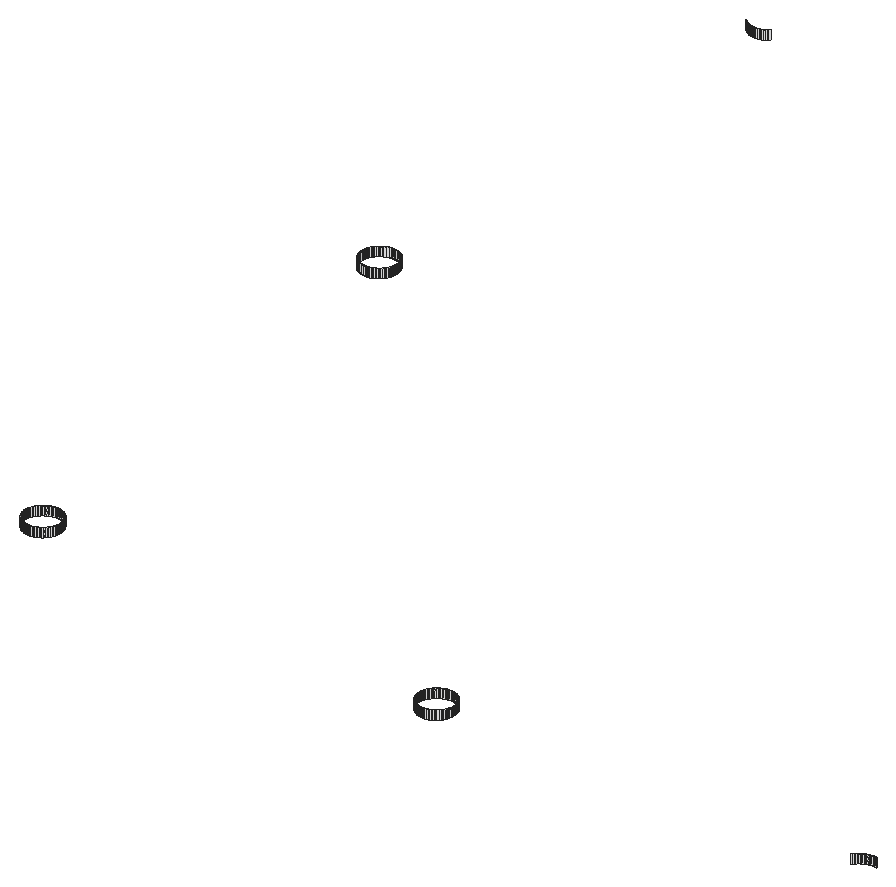
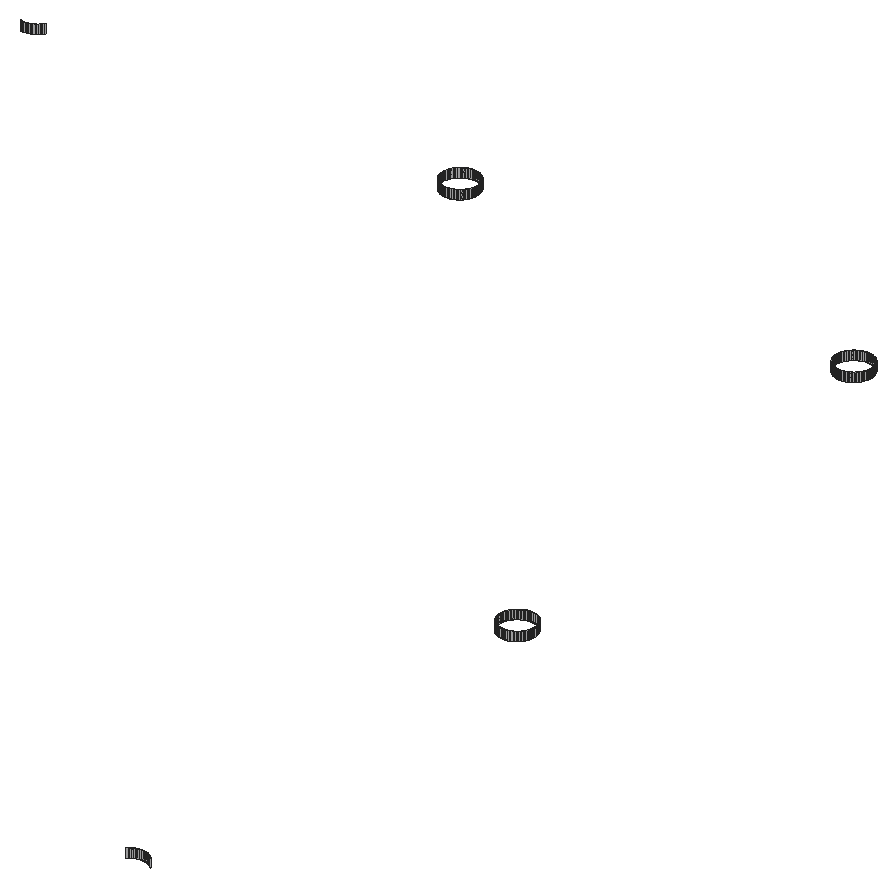
# SketchUp Ruby script. Lengths in inches.
U = 1.inch
M = Sketchup.active_model
def pt(a) = Geom::Point3d.new(a.map { |v| v * U })
def face(e, loops, mat)
  f = e.add_face(loops[0].map { |a| pt(a) })
  loops[1..].each { |l| e.add_face(l.map { |a| pt(a) }).erase! }
  f.material = f.back_material = mat if mat
  f
end
# faces: each face lists its corners as indices into pts; further lists are holes
def faces(e, pts, list, mat = nil) = list.each { |f| face(e, (f[0].is_a?(Array) ? f : [f]).map { |l| l.map { |i| pts[i] } }, mat) }
# xy, xz, yz: faces in a plane at the given z, y or x. An outline is a flat list of corners, or four numbers for a rectangle; further outlines are holes
def ring(l) = l.size == 4 ? [[l[0], l[1]], [l[2], l[1]], [l[2], l[3]], [l[0], l[3]]] : l.each_slice(2).to_a
def flat(e, list, mat, &to3) = list.each { |f| face(e, (f[0].is_a?(Array) ? f : [f]).map { |l| ring(l).map { |u, v| to3.(u, v) } }, mat) }
def xy(e, z, list, mat = nil) = flat(e, list, mat) { |x, y| [x, y, z] }
def xz(e, y, list, mat = nil) = flat(e, list, mat) { |x, z| [x, y, z] }
def yz(e, x, list, mat = nil) = flat(e, list, mat) { |y, z| [x, y, z] }
def lines(e, pts, list) = list.each { |a, b| e.add_line(pt(pts[a]), pt(pts[b])) }
# prism: a flat outline (further loops are holes) pulled along v
def prism(e, loops, v, mat = nil)
  f = face(e, loops, mat); d = Geom::Vector3d.new(v.map { |x| x * U })
  f.pushpull(f.normal.samedirection?(d) ? d.length : -d.length)
end
def box(e, o, s, mat = nil) = prism(e, [[o, [o[0] + s[0], o[1], o[2]], [o[0] + s[0], o[1] + s[1], o[2]], [o[0], o[1] + s[1], o[2]]]], [0, 0, s[2]], mat)
def at(x, y, z, deg = 0) = Geom::Transformation.translation(pt([x, y, z])) * Geom::Transformation.rotation(ORIGIN, Z_AXIS, deg.degrees)
def axes(o, x, y, z) = Geom::Transformation.new([*x, 0, *y, 0, *z, 0, *pt(o).to_a, 1])
def part(name) = M.definitions.add(name)
# library, detail: a bought-in or finely detailed component or shape, given as its bounding box
def library(name, o, s) = part(name).tap { |d| box(d.entities, o, s) }
def detail(e, o, s) = box(e.add_group.entities, o, s)
def put(e, d, t, mat = nil) = e.add_instance(d, t).tap { |i| i.material = mat if mat }
def group(e, t, mat = nil) = e.add_group.tap { |g| g.transformation = t; g.material = mat if mat }.entities
root = M.entities
M.materials.add("[Quartz Light Grey]").color = [251, 251, 252]
xz(root,52,[[86.9,111.81,87.02,112.81]],"[Quartz Light Grey]")
xz(root,56,[[38.9,111.81,39.02,112.81],[86.98,111.81,87.1,112.81],[134.98,111.81,135.1,112.81]],"[Quartz Light Grey]")
xz(root,60,[[38.98,111.81,39.1,112.81]],"[Quartz Light Grey]")
xz(root,115.35,[[32.85,111.81,32.98,112.81],[32.98,111.81,33.1,112.81]],"[Quartz Light Grey]")
xz(root,166.71,[[32.9,111.81,33.02,112.81],[33.02,111.81,33.15,112.81]],"[Quartz Light Grey]")
yz(root,31,[[113.33,111.81,113.46,112.81]],"[Quartz Light Grey]")
yz(root,35,[[113.25,111.81,113.375,112.81]],"[Quartz Light Grey]")
yz(root,37,[[57.98,111.81,58.1,112.81]],"[Quartz Light Grey]")
yz(root,41,[[57.9,111.81,58.02,112.81]],"[Quartz Light Grey]")
yz(root,85,[[53.98,111.81,54.1,112.81]],"[Quartz Light Grey]")
yz(root,89,[[53.9,111.81,54.02,112.81]],"[Quartz Light Grey]")
p = [[86.65,52.03,111.81],[86.52,52.06,111.81],[86.52,52.06,112.81],[86.65,52.03,112.81],[86.77,52.01,111.81],[86.77,52.01,112.81],
  [86.9,52,111.81],[86.9,52,112.81],[87.15,52.01,111.81],[87.02,52,111.81],[87.02,52,112.81],[87.15,52.01,112.81],
  [87.27,52.02,111.81],[87.27,52.02,112.81],[87.4,52.04,111.81],[87.4,52.04,112.81],[87.52,52.07,111.81],[87.52,52.07,112.81],
  [86.28,52.13,111.81],[86.17,52.18,111.81],[86.17,52.18,112.81],[86.28,52.13,112.81],[86.4,52.09,111.81],[86.4,52.09,112.81],
  [87.64,52.1,111.81],[87.64,52.1,112.81],[87.76,52.15,111.81],[87.76,52.15,112.81],[87.87,52.2,111.81],[87.87,52.2,112.81],
  [86.06,52.24,111.81],[85.95,52.3,111.81],[85.95,52.3,112.81],[86.06,52.24,112.81],[87.98,52.26,111.81],[87.98,52.26,112.81],
  [85.84,52.37,111.81],[85.84,52.37,112.81],[88.09,52.32,111.81],[88.09,52.32,112.81],[88.19,52.39,111.81],[88.19,52.39,112.81],
  [85.74,52.45,111.81],[85.65,52.53,111.81],[85.65,52.53,112.81],[85.74,52.45,112.81],[88.29,52.47,111.81],[88.29,52.47,112.81],
  [85.56,52.62,111.81],[85.56,52.62,112.81],[88.38,52.56,111.81],[88.38,52.56,112.81],[85.47,52.71,111.81],[85.47,52.71,112.81],
  [88.47,52.65,111.81],[88.47,52.65,112.81],[88.55,52.74,111.81],[88.55,52.74,112.81],[85.39,52.81,111.81],[85.39,52.81,112.81],
  [88.63,52.84,111.81],[88.63,52.84,112.81],[85.32,52.91,111.81],[85.32,52.91,112.81],[88.7,52.95,111.81],[88.7,52.95,112.81],
  [85.26,53.02,111.81],[85.26,53.02,112.81],[88.76,53.06,111.81],[88.76,53.06,112.81],[85.2,53.13,111.81],[85.2,53.13,112.81],
  [85.15,53.24,111.81],[85.15,53.24,112.81],[88.82,53.17,111.81],[88.82,53.17,112.81],[85.1,53.36,111.81],[85.1,53.36,112.81],
  [88.87,53.28,111.81],[88.87,53.28,112.81],[88.91,53.4,111.81],[88.91,53.4,112.81],[85.07,53.48,111.81],[85.07,53.48,112.81],
  [88.94,53.52,111.81],[88.94,53.52,112.81],[85.04,53.6,111.81],[85.04,53.6,112.81],[88.97,53.65,111.81],[88.97,53.65,112.81],
  [85.02,53.73,111.81],[85.02,53.73,112.81],[88.99,53.77,111.81],[88.99,53.77,112.81],[85.01,53.85,111.81],[85.01,53.85,112.81],
  [89,53.9,111.81],[89,53.9,112.81],[85,53.98,111.81],[85,53.98,112.81],[88.99,54.15,111.81],[89,54.02,111.81],
  [89,54.02,112.81],[88.99,54.15,112.81],[85,54.1,111.81],[85.01,54.23,111.81],[85.01,54.23,112.81],[85,54.1,112.81],
  [88.98,54.27,111.81],[88.98,54.27,112.81],[85.03,54.35,111.81],[85.03,54.35,112.81],[88.96,54.4,111.81],[88.96,54.4,112.81],
  [85.06,54.48,111.81],[85.06,54.48,112.81],[88.93,54.52,111.81],[88.93,54.52,112.81],[85.09,54.6,111.81],[85.09,54.6,112.81],
  [88.9,54.64,111.81],[88.9,54.64,112.81],[85.13,54.72,111.81],[85.13,54.72,112.81],[88.85,54.76,111.81],[88.85,54.76,112.81],
  [85.18,54.83,111.81],[85.18,54.83,112.81],[85.24,54.94,111.81],[85.24,54.94,112.81],[88.8,54.87,111.81],[88.8,54.87,112.81],
  [85.3,55.05,111.81],[85.3,55.05,112.81],[88.74,54.98,111.81],[88.74,54.98,112.81],[88.68,55.09,111.81],[88.68,55.09,112.81],
  [85.37,55.16,111.81],[85.37,55.16,112.81],[88.61,55.19,111.81],[88.61,55.19,112.81],[133.3,55.05,111.81],[133.37,55.16,111.81],
  [133.37,55.16,112.81],[133.3,55.05,112.81],[85.45,55.26,111.81],[85.45,55.26,112.81],[88.53,55.29,111.81],[88.53,55.29,112.81],
  [133.45,55.26,111.81],[133.45,55.26,112.81],[85.53,55.35,111.81],[85.53,55.35,112.81],[88.44,55.38,111.81],[88.44,55.38,112.81],
  [133.53,55.35,111.81],[133.53,55.35,112.81],[85.62,55.44,111.81],[85.62,55.44,112.81],[85.71,55.53,111.81],[85.71,55.53,112.81],
  [88.35,55.47,111.81],[88.35,55.47,112.81],[133.62,55.44,111.81],[133.62,55.44,112.81],[133.71,55.53,111.81],[133.71,55.53,112.81],
  [85.81,55.61,111.81],[85.81,55.61,112.81],[88.26,55.55,111.81],[88.26,55.55,112.81],[133.81,55.61,111.81],[133.81,55.61,112.81],
  [85.91,55.68,111.81],[85.91,55.68,112.81],[88.05,55.7,111.81],[88.16,55.63,111.81],[88.16,55.63,112.81],[88.05,55.7,112.81],
  [133.91,55.68,111.81],[133.91,55.68,112.81],[86.02,55.74,111.81],[86.02,55.74,112.81],[86.13,55.8,111.81],[86.13,55.8,112.81],
  [87.94,55.76,111.81],[87.94,55.76,112.81],[134.02,55.74,111.81],[134.02,55.74,112.81],[134.13,55.8,111.81],[134.13,55.8,112.81],
  [86.24,55.85,111.81],[86.24,55.85,112.81],[87.72,55.87,111.81],[87.83,55.82,111.81],[87.83,55.82,112.81],[87.72,55.87,112.81],
  [134.24,55.85,111.81],[134.24,55.85,112.81],[86.36,55.9,111.81],[86.36,55.9,112.81],[86.48,55.93,111.81],[86.48,55.93,112.81],
  [86.6,55.96,111.81],[86.6,55.96,112.81],[87.35,55.97,111.81],[87.48,55.94,111.81],[87.48,55.94,112.81],[87.35,55.97,112.81],
  [87.6,55.91,111.81],[87.6,55.91,112.81],[134.36,55.9,111.81],[134.36,55.9,112.81],[134.48,55.93,111.81],[134.48,55.93,112.81],
  [134.6,55.96,111.81],[134.6,55.96,112.81],[135.35,55.97,111.81],[135.48,55.94,111.81],[135.48,55.94,112.81],[135.35,55.97,112.81],
  [38.65,56.03,111.81],[38.52,56.06,111.81],[38.52,56.06,112.81],[38.65,56.03,112.81],[38.77,56.01,111.81],[38.77,56.01,112.81],
  [38.9,56,111.81],[38.9,56,112.81],[39.15,56.01,111.81],[39.02,56,111.81],[39.02,56,112.81],[39.15,56.01,112.81],
  [39.27,56.02,111.81],[39.27,56.02,112.81],[39.4,56.04,111.81],[39.4,56.04,112.81],[39.52,56.07,111.81],[39.52,56.07,112.81],
  [86.73,55.98,111.81],[86.73,55.98,112.81],[86.85,55.99,111.81],[86.85,55.99,112.81],[86.98,56,111.81],[86.98,56,112.81],
  [87.1,56,111.81],[87.23,55.99,111.81],[87.23,55.99,112.81],[87.1,56,112.81],[134.73,55.98,111.81],[134.73,55.98,112.81],
  [134.85,55.99,111.81],[134.85,55.99,112.81],[134.98,56,111.81],[134.98,56,112.81],[135.1,56,111.81],[135.23,55.99,111.81],
  [135.23,55.99,112.81],[135.1,56,112.81],[38.28,56.13,111.81],[38.17,56.18,111.81],[38.17,56.18,112.81],[38.28,56.13,112.81],
  [38.4,56.09,111.81],[38.4,56.09,112.81],[39.64,56.1,111.81],[39.64,56.1,112.81],[39.76,56.15,111.81],[39.76,56.15,112.81],
  [39.87,56.2,111.81],[39.87,56.2,112.81],[38.06,56.24,111.81],[37.95,56.3,111.81],[37.95,56.3,112.81],[38.06,56.24,112.81],
  [39.98,56.26,111.81],[39.98,56.26,112.81],[37.84,56.37,111.81],[37.84,56.37,112.81],[40.09,56.32,111.81],[40.09,56.32,112.81],
  [40.19,56.39,111.81],[40.19,56.39,112.81],[37.74,56.45,111.81],[37.65,56.53,111.81],[37.65,56.53,112.81],[37.74,56.45,112.81],
  [40.29,56.47,111.81],[40.29,56.47,112.81],[37.56,56.62,111.81],[37.56,56.62,112.81],[40.38,56.56,111.81],[40.38,56.56,112.81],
  [37.47,56.71,111.81],[37.47,56.71,112.81],[40.47,56.65,111.81],[40.47,56.65,112.81],[40.55,56.74,111.81],[40.55,56.74,112.81],
  [37.39,56.81,111.81],[37.39,56.81,112.81],[40.63,56.84,111.81],[40.63,56.84,112.81],[37.32,56.91,111.81],[37.32,56.91,112.81],
  [40.7,56.95,111.81],[40.7,56.95,112.81],[37.26,57.02,111.81],[37.26,57.02,112.81],[40.76,57.06,111.81],[40.76,57.06,112.81],
  [37.2,57.13,111.81],[37.2,57.13,112.81],[37.15,57.24,111.81],[37.15,57.24,112.81],[40.82,57.17,111.81],[40.82,57.17,112.81],
  [37.1,57.36,111.81],[37.1,57.36,112.81],[40.87,57.28,111.81],[40.87,57.28,112.81],[40.91,57.4,111.81],[40.91,57.4,112.81],
  [37.07,57.48,111.81],[37.07,57.48,112.81],[40.94,57.52,111.81],[40.94,57.52,112.81],[37.04,57.6,111.81],[37.04,57.6,112.81],
  [40.97,57.65,111.81],[40.97,57.65,112.81],[37.02,57.73,111.81],[37.02,57.73,112.81],[40.99,57.77,111.81],[40.99,57.77,112.81],
  [37.01,57.85,111.81],[37.01,57.85,112.81],[41,57.9,111.81],[41,57.9,112.81],[37,57.98,111.81],[37,57.98,112.81],
  [40.99,58.15,111.81],[41,58.02,111.81],[41,58.02,112.81],[40.99,58.15,112.81],[37,58.1,111.81],[37.01,58.23,111.81],
  [37.01,58.23,112.81],[37,58.1,112.81],[40.98,58.27,111.81],[40.98,58.27,112.81],[37.03,58.35,111.81],[37.03,58.35,112.81],
  [40.96,58.4,111.81],[40.96,58.4,112.81],[37.06,58.48,111.81],[37.06,58.48,112.81],[40.93,58.52,111.81],[40.93,58.52,112.81],
  [37.09,58.6,111.81],[37.09,58.6,112.81],[40.9,58.64,111.81],[40.9,58.64,112.81],[37.13,58.72,111.81],[37.13,58.72,112.81],
  [40.85,58.76,111.81],[40.85,58.76,112.81],[37.18,58.83,111.81],[37.18,58.83,112.81],[37.24,58.94,111.81],[37.24,58.94,112.81],
  [40.8,58.87,111.81],[40.8,58.87,112.81],[37.3,59.05,111.81],[37.3,59.05,112.81],[40.74,58.98,111.81],[40.74,58.98,112.81],
  [40.68,59.09,111.81],[40.68,59.09,112.81],[37.37,59.16,111.81],[37.37,59.16,112.81],[40.61,59.19,111.81],[40.61,59.19,112.81],
  [37.45,59.26,111.81],[37.45,59.26,112.81],[40.53,59.29,111.81],[40.53,59.29,112.81],[37.53,59.35,111.81],[37.53,59.35,112.81],
  [40.44,59.38,111.81],[40.44,59.38,112.81],[37.62,59.44,111.81],[37.62,59.44,112.81],[37.71,59.53,111.81],[37.71,59.53,112.81],
  [40.35,59.47,111.81],[40.35,59.47,112.81],[37.81,59.61,111.81],[37.81,59.61,112.81],[40.26,59.55,111.81],[40.26,59.55,112.81],
  [37.91,59.68,111.81],[37.91,59.68,112.81],[40.05,59.7,111.81],[40.16,59.63,111.81],[40.16,59.63,112.81],[40.05,59.7,112.81],
  [38.02,59.74,111.81],[38.02,59.74,112.81],[38.13,59.8,111.81],[38.13,59.8,112.81],[39.94,59.76,111.81],[39.94,59.76,112.81],
  [38.24,59.85,111.81],[38.24,59.85,112.81],[39.72,59.87,111.81],[39.83,59.82,111.81],[39.83,59.82,112.81],[39.72,59.87,112.81],
  [38.36,59.9,111.81],[38.36,59.9,112.81],[38.48,59.93,111.81],[38.48,59.93,112.81],[38.6,59.96,111.81],[38.6,59.96,112.81],
  [39.35,59.97,111.81],[39.48,59.94,111.81],[39.48,59.94,112.81],[39.35,59.97,112.81],[39.6,59.91,111.81],[39.6,59.91,112.81],
  [38.73,59.98,111.81],[38.73,59.98,112.81],[38.85,59.99,111.81],[38.85,59.99,112.81],[38.98,60,111.81],[38.98,60,112.81],
  [39.1,60,111.81],[39.23,59.99,111.81],[39.23,59.99,112.81],[39.1,60,112.81],[32.4,111.45,111.81],[32.28,111.49,111.81],
  [32.28,111.49,112.81],[32.4,111.45,112.81],[32.52,111.41,111.81],[32.52,111.41,112.81],[32.65,111.39,111.81],[32.65,111.39,112.81],
  [32.77,111.37,111.81],[32.77,111.37,112.81],[32.9,111.36,111.81],[32.9,111.36,112.81],[33.02,111.35,111.81],[33.02,111.35,112.81],
  [33.15,111.36,111.81],[33.15,111.36,112.81],[33.27,111.37,111.81],[33.27,111.37,112.81],[33.4,111.39,111.81],[33.4,111.39,112.81],
  [33.52,111.42,111.81],[33.52,111.42,112.81],[33.64,111.46,111.81],[33.64,111.46,112.81],[32.17,111.54,111.81],[32.06,111.59,111.81],
  [32.06,111.59,112.81],[32.17,111.54,112.81],[33.76,111.5,111.81],[33.76,111.5,112.81],[33.87,111.55,111.81],[33.87,111.55,112.81],
  [31.95,111.65,111.81],[31.95,111.65,112.81],[33.98,111.61,111.81],[33.98,111.61,112.81],[34.09,111.68,111.81],[34.09,111.68,112.81],
  [31.84,111.72,111.81],[31.74,111.8,111.81],[31.74,111.8,112.81],[31.84,111.72,112.81],[34.19,111.75,111.81],[34.19,111.75,112.81],
  [34.29,111.83,111.81],[34.29,111.83,112.81],[31.65,111.88,111.81],[31.65,111.88,112.81],[34.38,111.91,111.81],[34.38,111.91,112.81],
  [31.56,111.97,111.81],[31.56,111.97,112.81],[34.47,112,111.81],[34.47,112,112.81],[31.47,112.0625,111.81],[31.47,112.0625,112.81],
  [34.55,112.1,111.81],[34.55,112.1,112.81],[31.39,112.16,111.81],[31.39,112.16,112.81],[34.63,112.2,111.81],[34.63,112.2,112.81],
  [31.32,112.26,111.81],[31.32,112.26,112.81],[34.7,112.3,111.81],[34.7,112.3,112.81],[31.26,112.37,111.81],[31.26,112.37,112.81],
  [34.76,112.41,111.81],[34.76,112.41,112.81],[31.2,112.48,111.81],[31.2,112.48,112.81],[34.82,112.52,111.81],[34.82,112.52,112.81],
  [31.15,112.6,111.81],[31.15,112.6,112.81],[34.87,112.64,111.81],[34.87,112.64,112.81],[31.1,112.72,111.81],[31.1,112.72,112.81],
  [34.91,112.76,111.81],[34.91,112.76,112.81],[31.07,112.84,111.81],[31.07,112.84,112.81],[31.04,112.96,111.81],[31.04,112.96,112.81],
  [34.94,112.88,111.81],[34.94,112.88,112.81],[34.97,113,111.81],[34.97,113,112.81],[31.02,113.08,111.81],[31.02,113.08,112.81],
  [34.99,113.125,111.81],[34.99,113.125,112.81],[31.01,113.21,111.81],[31.01,113.21,112.81],[35,113.25,111.81],[35,113.25,112.81],
  [31,113.33,111.81],[31,113.33,112.81],[34.99,113.5,111.81],[35,113.375,111.81],[35,113.375,112.81],[34.99,113.5,112.81],
  [31,113.46,111.81],[31.01,113.58,111.81],[31.01,113.58,112.81],[31,113.46,112.81],[34.98,113.625,111.81],[34.98,113.625,112.81],
  [31.03,113.71,111.81],[31.03,113.71,112.81],[34.96,113.75,111.81],[34.96,113.75,112.81],[31.06,113.83,111.81],[31.06,113.83,112.81],
  [31.09,113.95,111.81],[31.09,113.95,112.81],[34.93,113.87,111.81],[34.93,113.87,112.81],[34.9,113.99,111.81],[34.9,113.99,112.81],
  [31.13,114.07,111.81],[31.13,114.07,112.81],[34.85,114.11,111.81],[34.85,114.11,112.81],[31.18,114.1875,111.81],[31.18,114.1875,112.81],
  [34.8,114.23,111.81],[34.8,114.23,112.81],[31.24,114.3,111.81],[31.24,114.3,112.81],[34.74,114.34,111.81],[34.74,114.34,112.81],
  [31.3,114.41,111.81],[31.3,114.41,112.81],[34.68,114.44,111.81],[34.68,114.44,112.81],[31.37,114.51,111.81],[31.37,114.51,112.81],
  [34.61,114.55,111.81],[34.61,114.55,112.81],[31.45,114.61,111.81],[31.45,114.61,112.81],[34.53,114.65,111.81],[34.53,114.65,112.81],
  [31.53,114.71,111.81],[31.53,114.71,112.81],[34.44,114.74,111.81],[34.44,114.74,112.81],[31.62,114.8,111.81],[31.62,114.8,112.81],
  [34.35,114.83,111.81],[34.35,114.83,112.81],[31.71,114.88,111.81],[31.71,114.88,112.81],[34.26,114.91,111.81],[34.26,114.91,112.81],
  [31.81,114.96,111.81],[31.81,114.96,112.81],[34.16,114.98,111.81],[34.16,114.98,112.81],[31.91,115.03,111.81],[31.91,115.03,112.81],
  [32.02,115.1,111.81],[32.02,115.1,112.81],[34.05,115.05,111.81],[34.05,115.05,112.81],[32.13,115.15,111.81],[32.13,115.15,112.81],
  [33.83,115.17,111.81],[33.94,115.12,111.81],[33.94,115.12,112.81],[33.83,115.17,112.81],[32.24,115.21,111.81],[32.24,115.21,112.81],
  [32.36,115.25,111.81],[32.36,115.25,112.81],[32.48,115.29,111.81],[32.48,115.29,112.81],[33.6,115.26,111.81],[33.72,115.22,111.81],
  [33.72,115.22,112.81],[33.6,115.26,112.81],[32.6,115.31,111.81],[32.6,115.31,112.81],[32.73,115.34,111.81],[32.73,115.34,112.81],
  [32.85,115.35,111.81],[32.85,115.35,112.81],[33.1,115.35,111.81],[33.23,115.34,111.81],[33.23,115.34,112.81],[33.1,115.35,112.81],
  [33.35,115.32,111.81],[33.35,115.32,112.81],[33.48,115.3,111.81],[33.48,115.3,112.81],[32.65,166.74,111.81],[32.52,166.77,111.81],
  [32.52,166.77,112.81],[32.65,166.74,112.81],[32.77,166.72,111.81],[32.77,166.72,112.81],[32.9,166.71,111.81],[32.9,166.71,112.81],
  [33.27,166.73,111.81],[33.15,166.71,111.81],[33.15,166.71,112.81],[33.27,166.73,112.81],[33.4,166.75,111.81],[33.4,166.75,112.81],
  [33.52,166.78,111.81],[33.52,166.78,112.81],[32.28,166.84,111.81],[32.17,166.89,111.81],[32.17,166.89,112.81],[32.28,166.84,112.81],
  [32.4,166.8,111.81],[32.4,166.8,112.81],[33.64,166.8125,111.81],[33.64,166.8125,112.81],[33.76,166.86,111.81],[33.76,166.86,112.81],
  [32.06,166.95,111.81],[31.95,167.01,111.81],[31.95,167.01,112.81],[32.06,166.95,112.81],[33.87,166.91,111.81],[33.87,166.91,112.81],
  [33.98,166.97,111.81],[33.98,166.97,112.81],[31.84,167.08,111.81],[31.84,167.08,112.81],[34.09,167.03,111.81],[34.09,167.03,112.81],
  [34.19,167.1,111.81],[34.19,167.1,112.81],[31.74,167.15,111.81],[31.74,167.15,112.81],[34.29,167.18,111.81],[34.29,167.18,112.81],
  [31.65,167.24,111.81],[31.65,167.24,112.81],[31.56,167.32,111.81],[31.56,167.32,112.81],[34.38,167.27,111.81],[34.38,167.27,112.81]]
faces(root,p,[[0,1,2,3],[4,0,3,5],[6,4,5,7],[8,9,10,11],[12,8,11,13],[14,12,13,15],[16,14,15,17],[18,19,20,21],
  [22,18,21,23],[1,22,23,2],[24,16,17,25],[26,24,25,27],[28,26,27,29],[30,31,32,33],[19,30,33,20],[34,28,29,35],
  [31,36,37,32],[38,34,35,39],[40,38,39,41],[42,43,44,45],[36,42,45,37],[46,40,41,47],[43,48,49,44],[50,46,47,51],
  [48,52,53,49],[54,50,51,55],[56,54,55,57],[52,58,59,53],[60,56,57,61],[58,62,63,59],[64,60,61,65],[62,66,67,63],
  [68,64,65,69],[66,70,71,67],[70,72,73,71],[74,68,69,75],[72,76,77,73],[78,74,75,79],[80,78,79,81],[76,82,83,77],
  [84,80,81,85],[82,86,87,83],[88,84,85,89],[86,90,91,87],[92,88,89,93],[90,94,95,91],[96,92,93,97],[94,98,99,95],
  [100,101,102,103],[104,105,106,107],[108,100,103,109],[105,110,111,106],[112,108,109,113],[110,114,115,111],[116,112,113,117],[114,118,119,115],
  [120,116,117,121],[118,122,123,119],[124,120,121,125],[122,126,127,123],[126,128,129,127],[130,124,125,131],[128,132,133,129],[134,130,131,135],
  [136,134,135,137],[132,138,139,133],[140,136,137,141],[142,143,144,145],[138,146,147,139],[148,140,141,149],[143,150,151,144],[146,152,153,147],
  [154,148,149,155],[150,156,157,151],[152,158,159,153],[158,160,161,159],[162,154,155,163],[156,164,165,157],[164,166,167,165],[160,168,169,161],
  [170,162,163,171],[166,172,173,167],[168,174,175,169],[176,177,178,179],[177,170,171,178],[172,180,181,173],[174,182,183,175],[182,184,185,183],
  [186,176,179,187],[180,188,189,181],[188,190,191,189],[184,192,193,185],[194,195,196,197],[195,186,187,196],[190,198,199,191],[192,200,201,193],
  [200,202,203,201],[202,204,205,203],[206,207,208,209],[207,210,211,208],[210,194,197,211],[198,212,213,199],[212,214,215,213],[214,216,217,215],
  [218,219,220,221],[222,223,224,225],[226,222,225,227],[228,226,227,229],[230,231,232,233],[234,230,233,235],[236,234,235,237],[238,236,237,239],
  [204,240,241,205],[240,242,243,241],[242,244,245,243],[246,247,248,249],[247,206,209,248],[216,250,251,217],[250,252,253,251],[252,254,255,253],
  [256,257,258,259],[257,218,221,258],[260,261,262,263],[264,260,263,265],[223,264,265,224],[266,238,239,267],[268,266,267,269],[270,268,269,271],
  [272,273,274,275],[261,272,275,262],[276,270,271,277],[273,278,279,274],[280,276,277,281],[282,280,281,283],[284,285,286,287],[278,284,287,279],
  [288,282,283,289],[285,290,291,286],[292,288,289,293],[290,294,295,291],[296,292,293,297],[298,296,297,299],[294,300,301,295],[302,298,299,303],
  [300,304,305,301],[306,302,303,307],[304,308,309,305],[310,306,307,311],[308,312,313,309],[312,314,315,313],[316,310,311,317],[314,318,319,315],
  [320,316,317,321],[322,320,321,323],[318,324,325,319],[326,322,323,327],[324,328,329,325],[330,326,327,331],[328,332,333,329],[334,330,331,335],
  [332,336,337,333],[338,334,335,339],[336,340,341,337],[342,343,344,345],[346,347,348,349],[350,342,345,351],[347,352,353,348],[354,350,351,355],
  [352,356,357,353],[358,354,355,359],[356,360,361,357],[362,358,359,363],[360,364,365,361],[366,362,363,367],[364,368,369,365],[368,370,371,369],
  [372,366,367,373],[370,374,375,371],[376,372,373,377],[378,376,377,379],[374,380,381,375],[382,378,379,383],[380,384,385,381],[386,382,383,387],
  [384,388,389,385],[390,386,387,391],[388,392,393,389],[392,394,395,393],[396,390,391,397],[394,398,399,395],[400,396,397,401],[398,402,403,399],
  [404,405,406,407],[405,400,401,406],[402,408,409,403],[408,410,411,409],[412,404,407,413],[410,414,415,411],[416,417,418,419],[417,412,413,418],
  [414,420,421,415],[420,422,423,421],[422,424,425,423],[426,427,428,429],[427,430,431,428],[430,416,419,431],[424,432,433,425],[432,434,435,433],
  [434,436,437,435],[438,439,440,441],[439,426,429,440],[442,443,444,445],[446,442,445,447],[448,446,447,449],[450,448,449,451],[452,450,451,453],
  [454,452,453,455],[456,454,455,457],[458,456,457,459],[460,458,459,461],[462,460,461,463],[464,462,463,465],[466,467,468,469],[443,466,469,444],
  [470,464,465,471],[472,470,471,473],[467,474,475,468],[476,472,473,477],[478,476,477,479],[480,481,482,483],[474,480,483,475],[484,478,479,485],
  [486,484,485,487],[481,488,489,482],[490,486,487,491],[488,492,493,489],[494,490,491,495],[492,496,497,493],[498,494,495,499],[496,500,501,497],
  [502,498,499,503],[500,504,505,501],[506,502,503,507],[504,508,509,505],[510,506,507,511],[508,512,513,509],[514,510,511,515],[512,516,517,513],
  [518,514,515,519],[516,520,521,517],[522,518,519,523],[520,524,525,521],[524,526,527,525],[528,522,523,529],[530,528,529,531],[526,532,533,527],
  [534,530,531,535],[532,536,537,533],[538,534,535,539],[536,540,541,537],[542,543,544,545],[546,547,548,549],[550,542,545,551],[547,552,553,548],
  [554,550,551,555],[552,556,557,553],[556,558,559,557],[560,554,555,561],[562,560,561,563],[558,564,565,559],[566,562,563,567],[564,568,569,565],
  [570,566,567,571],[568,572,573,569],[574,570,571,575],[572,576,577,573],[578,574,575,579],[576,580,581,577],[582,578,579,583],[580,584,585,581],
  [586,582,583,587],[584,588,589,585],[590,586,587,591],[588,592,593,589],[594,590,591,595],[592,596,597,593],[598,594,595,599],[596,600,601,597],
  [602,598,599,603],[600,604,605,601],[604,606,607,605],[608,602,603,609],[606,610,611,607],[612,613,614,615],[613,608,609,614],[610,616,617,611],
  [616,618,619,617],[618,620,621,619],[622,623,624,625],[623,612,615,624],[620,626,627,621],[626,628,629,627],[628,630,631,629],[632,633,634,635],
  [633,636,637,634],[636,638,639,637],[638,622,625,639],[640,641,642,643],[644,640,643,645],[646,644,645,647],[648,649,650,651],[652,648,651,653],
  [654,652,653,655],[656,657,658,659],[660,656,659,661],[641,660,661,642],[662,654,655,663],[664,662,663,665],[666,667,668,669],[657,666,669,658],
  [670,664,665,671],[672,670,671,673],[667,674,675,668],[676,672,673,677],[678,676,677,679],[674,680,681,675],[682,678,679,683],[680,684,685,681],
  [684,686,687,685],[688,682,683,689]],"[Quartz Light Grey]")
